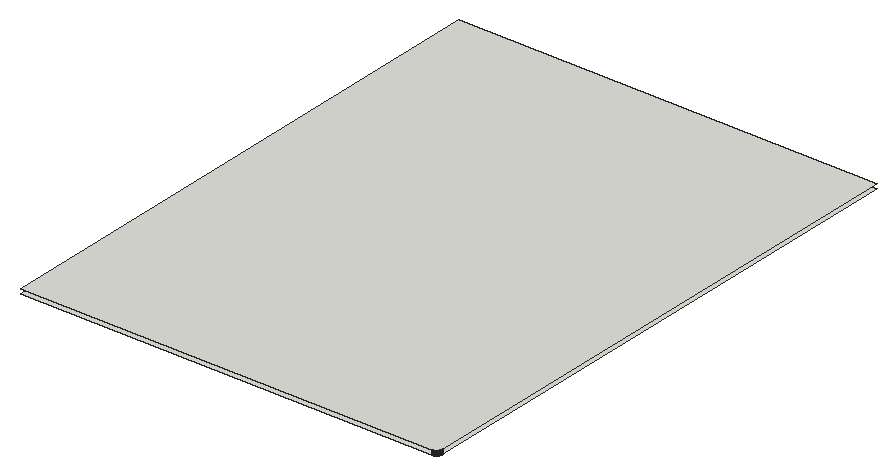
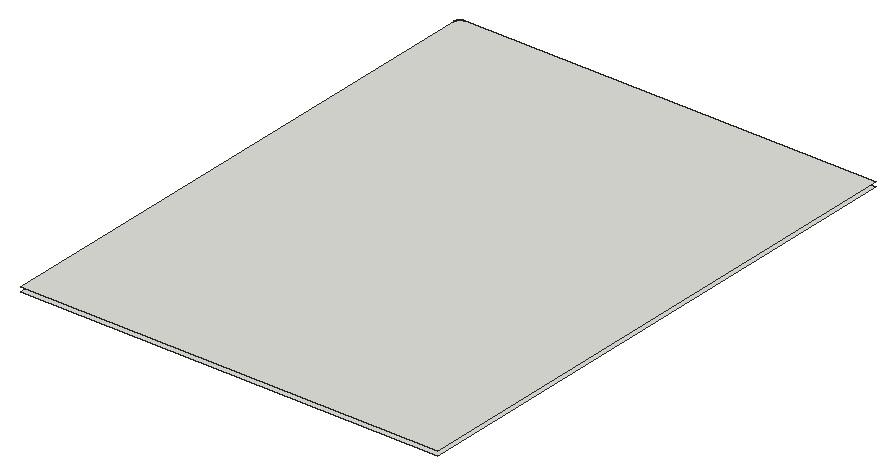
# SketchUp Ruby script. Lengths in inches.
U = 1.inch
M = Sketchup.active_model
def pt(a) = Geom::Point3d.new(a.map { |v| v * U })
def face(e, loops, mat)
  f = e.add_face(loops[0].map { |a| pt(a) })
  loops[1..].each { |l| e.add_face(l.map { |a| pt(a) }).erase! }
  f.material = f.back_material = mat if mat
  f
end
# faces: each face lists its corners as indices into pts; further lists are holes
def faces(e, pts, list, mat = nil) = list.each { |f| face(e, (f[0].is_a?(Array) ? f : [f]).map { |l| l.map { |i| pts[i] } }, mat) }
# xy, xz, yz: faces in a plane at the given z, y or x. An outline is a flat list of corners, or four numbers for a rectangle; further outlines are holes
def ring(l) = l.size == 4 ? [[l[0], l[1]], [l[2], l[1]], [l[2], l[3]], [l[0], l[3]]] : l.each_slice(2).to_a
def flat(e, list, mat, &to3) = list.each { |f| face(e, (f[0].is_a?(Array) ? f : [f]).map { |l| ring(l).map { |u, v| to3.(u, v) } }, mat) }
def xy(e, z, list, mat = nil) = flat(e, list, mat) { |x, y| [x, y, z] }
def xz(e, y, list, mat = nil) = flat(e, list, mat) { |x, z| [x, y, z] }
def yz(e, x, list, mat = nil) = flat(e, list, mat) { |y, z| [x, y, z] }
def lines(e, pts, list) = list.each { |a, b| e.add_line(pt(pts[a]), pt(pts[b])) }
# prism: a flat outline (further loops are holes) pulled along v
def prism(e, loops, v, mat = nil)
  f = face(e, loops, mat); d = Geom::Vector3d.new(v.map { |x| x * U })
  f.pushpull(f.normal.samedirection?(d) ? d.length : -d.length)
end
def box(e, o, s, mat = nil) = prism(e, [[o, [o[0] + s[0], o[1], o[2]], [o[0] + s[0], o[1] + s[1], o[2]], [o[0], o[1] + s[1], o[2]]]], [0, 0, s[2]], mat)
def at(x, y, z, deg = 0) = Geom::Transformation.translation(pt([x, y, z])) * Geom::Transformation.rotation(ORIGIN, Z_AXIS, deg.degrees)
def axes(o, x, y, z) = Geom::Transformation.new([*x, 0, *y, 0, *z, 0, *pt(o).to_a, 1])
def part(name) = M.definitions.add(name)
# library, detail: a bought-in or finely detailed component or shape, given as its bounding box
def library(name, o, s) = part(name).tap { |d| box(d.entities, o, s) }
def detail(e, o, s) = box(e.add_group.entities, o, s)
def put(e, d, t, mat = nil) = e.add_instance(d, t).tap { |i| i.material = mat if mat }
def group(e, t, mat = nil) = e.add_group.tap { |g| g.transformation = t; g.material = mat if mat }.entities
root = M.entities
xy(root,128,[[[48,96,48,600,432,600,432,101.78,431.95,101.23,431.93,101.12,431.92,101.01,431.9,100.9,431.85,100.68,431.83,100.57,431.8,100.46,431.77,100.36,431.74,100.25,431.71,100.15,431.67,100.04,431.63,99.9375,431.59,99.83,431.47,99.53,431.27,99.13,431.21,99.03,431.16,98.9375,431.1,98.84,430.98,98.66,430.92,98.5625,430.85,98.47,430.79,98.38,430.72,98.3,430.65,98.21,430.51,98.04,430.43,97.96,430.36,97.875,430.28,97.8,430.2,97.72,430.125,97.64,430.04,97.57,429.96,97.49,429.79,97.35,429.7,97.28,429.62,97.21,429.53,97.15,429.4375,97.08,429.34,97.02,429.16,96.9,429.0625,96.84,428.97,96.79,428.87,96.73,428.47,96.53,428.17,96.41,428.0625,96.37,427.96,96.33,427.85,96.29,427.75,96.26,427.64,96.23,427.54,96.2,427.43,96.17,427.32,96.15,427.1,96.1,426.99,96.08,426.88,96.07,426.77,96.05,426.22,96],[359.84,432,360.16,432,360.24,432.01,360.3125,432.02,360.39,432.03,360.55,432.05,360.625,432.07,360.7,432.08,360.78,432.1,360.85,432.125,360.93,432.15,361,432.17,361.08,432.2,361.29,432.29,361.36,432.33,361.43,432.36,361.57,432.44,361.63,432.48,361.7,432.53,361.76,432.57,361.83,432.62,362.07,432.82,362.12,432.88,362.18,432.93,362.38,433.17,362.43,433.24,362.47,433.3,362.52,433.37,362.56,433.43,362.64,433.57,362.67,433.64,362.71,433.71,362.8,433.92,362.83,434,362.85,434.07,362.875,434.15,362.9,434.22,362.92,434.3,362.93,434.375,362.95,434.45,362.97,434.61,362.98,434.6875,362.99,434.76,363,434.84,363,435.16,362.99,435.24,362.98,435.3125,362.97,435.39,362.95,435.55,362.93,435.625,362.92,435.7,362.9,435.78,362.875,435.85,362.85,435.93,362.83,436,362.8,436.08,362.71,436.29,362.67,436.36,362.64,436.43,362.56,436.57,362.52,436.63,362.47,436.7,362.43,436.76,362.38,436.83,362.18,437.07,362.12,437.12,362.07,437.18,361.83,437.38,361.76,437.43,361.7,437.47,361.63,437.52,361.57,437.56,361.43,437.64,361.36,437.67,361.29,437.71,361.08,437.8,361,437.83,360.93,437.85,360.85,437.875,360.78,437.9,360.7,437.92,360.625,437.93,360.55,437.95,360.39,437.97,360.3125,437.98,360.24,437.99,360.16,438,359.84,438,359.76,437.99,359.6875,437.98,359.61,437.97,359.45,437.95,359.375,437.93,359.3,437.92,359.22,437.9,359.15,437.875,359.07,437.85,359,437.83,358.92,437.8,358.71,437.71,358.64,437.67,358.57,437.64,358.43,437.56,358.37,437.52,358.3,437.47,358.24,437.43,358.17,437.38,357.93,437.18,357.88,437.12,357.82,437.07,357.62,436.83,357.57,436.76,357.53,436.7,357.48,436.63,357.44,436.57,357.36,436.43,357.33,436.36,357.29,436.29,357.2,436.08,357.17,436,357.15,435.93,357.125,435.85,357.1,435.78,357.08,435.7,357.07,435.625,357.05,435.55,357.03,435.39,357.02,435.3125,357.01,435.24,357,435.16,357,434.84,357.01,434.76,357.02,434.6875,357.03,434.61,357.05,434.45,357.07,434.375,357.08,434.3,357.1,434.22,357.125,434.15,357.15,434.07,357.17,434,357.2,433.92,357.29,433.71,357.33,433.64,357.36,433.57,357.44,433.43,357.48,433.37,357.53,433.3,357.57,433.24,357.62,433.17,357.82,432.93,357.88,432.88,357.93,432.82,358.17,432.62,358.24,432.57,358.3,432.53,358.37,432.48,358.43,432.44,358.57,432.36,358.64,432.33,358.71,432.29,358.92,432.2,359,432.17,359.07,432.15,359.15,432.125,359.22,432.1,359.3,432.08,359.375,432.07,359.45,432.05,359.61,432.03,359.6875,432.02,359.76,432.01],[359.84,525,360.16,525,360.24,525.01,360.3125,525.02,360.39,525.03,360.55,525.05,360.625,525.07,360.7,525.08,360.78,525.1,360.85,525.125,360.93,525.15,361,525.17,361.08,525.2,361.29,525.29,361.36,525.33,361.43,525.36,361.57,525.44,361.63,525.48,361.7,525.53,361.76,525.57,361.83,525.62,362.07,525.82,362.12,525.88,362.18,525.93,362.38,526.17,362.43,526.24,362.47,526.3,362.52,526.37,362.56,526.43,362.64,526.57,362.67,526.64,362.71,526.71,362.8,526.92,362.83,527,362.85,527.07,362.875,527.15,362.9,527.22,362.92,527.3,362.93,527.375,362.95,527.45,362.97,527.61,362.98,527.6875,362.99,527.76,363,527.84,363,528.16,362.99,528.24,362.98,528.3125,362.97,528.39,362.95,528.55,362.93,528.625,362.92,528.7,362.9,528.78,362.875,528.85,362.85,528.93,362.83,529,362.8,529.08,362.71,529.29,362.67,529.36,362.64,529.43,362.56,529.57,362.52,529.63,362.47,529.7,362.43,529.76,362.38,529.83,362.18,530.07,362.12,530.12,362.07,530.18,361.83,530.38,361.76,530.43,361.7,530.47,361.63,530.52,361.57,530.56,361.43,530.64,361.36,530.67,361.29,530.71,361.08,530.8,361,530.83,360.93,530.85,360.85,530.875,360.78,530.9,360.7,530.92,360.625,530.93,360.55,530.95,360.39,530.97,360.3125,530.98,360.24,530.99,360.16,531,359.84,531,359.76,530.99,359.6875,530.98,359.61,530.97,359.45,530.95,359.375,530.93,359.3,530.92,359.22,530.9,359.15,530.875,359.07,530.85,359,530.83,358.92,530.8,358.71,530.71,358.64,530.67,358.57,530.64,358.43,530.56,358.37,530.52,358.3,530.47,358.24,530.43,358.17,530.38,357.93,530.18,357.88,530.12,357.82,530.07,357.62,529.83,357.57,529.76,357.53,529.7,357.48,529.63,357.44,529.57,357.36,529.43,357.33,529.36,357.29,529.29,357.2,529.08,357.17,529,357.15,528.93,357.125,528.85,357.1,528.78,357.08,528.7,357.07,528.625,357.05,528.55,357.03,528.39,357.02,528.3125,357.01,528.24,357,528.16,357,527.84,357.01,527.76,357.02,527.6875,357.03,527.61,357.05,527.45,357.07,527.375,357.08,527.3,357.1,527.22,357.125,527.15,357.15,527.07,357.17,527,357.2,526.92,357.29,526.71,357.33,526.64,357.36,526.57,357.44,526.43,357.48,526.37,357.53,526.3,357.57,526.24,357.62,526.17,357.82,525.93,357.88,525.88,357.93,525.82,358.17,525.62,358.24,525.57,358.3,525.53,358.37,525.48,358.43,525.44,358.57,525.36,358.64,525.33,358.71,525.29,358.92,525.2,359,525.17,359.07,525.15,359.15,525.125,359.22,525.1,359.3,525.08,359.375,525.07,359.45,525.05,359.61,525.03,359.6875,525.02,359.76,525.01],[279.84,525,280.16,525,280.24,525.01,280.3125,525.02,280.39,525.03,280.55,525.05,280.625,525.07,280.7,525.08,280.78,525.1,280.85,525.125,280.93,525.15,281,525.17,281.08,525.2,281.29,525.29,281.36,525.33,281.43,525.36,281.57,525.44,281.63,525.48,281.7,525.53,281.76,525.57,281.83,525.62,282.07,525.82,282.12,525.88,282.18,525.93,282.38,526.17,282.43,526.24,282.47,526.3,282.52,526.37,282.56,526.43,282.64,526.57,282.67,526.64,282.71,526.71,282.8,526.92,282.83,527,282.85,527.07,282.875,527.15,282.9,527.22,282.92,527.3,282.93,527.375,282.95,527.45,282.97,527.61,282.98,527.6875,282.99,527.76,283,527.84,283,528.16,282.99,528.24,282.98,528.3125,282.97,528.39,282.95,528.55,282.93,528.625,282.92,528.7,282.9,528.78,282.875,528.85,282.85,528.93,282.83,529,282.8,529.08,282.71,529.29,282.67,529.36,282.64,529.43,282.56,529.57,282.52,529.63,282.47,529.7,282.43,529.76,282.38,529.83,282.18,530.07,282.12,530.12,282.07,530.18,281.83,530.38,281.76,530.43,281.7,530.47,281.63,530.52,281.57,530.56,281.43,530.64,281.36,530.67,281.29,530.71,281.08,530.8,281,530.83,280.93,530.85,280.85,530.875,280.78,530.9,280.7,530.92,280.625,530.93,280.55,530.95,280.39,530.97,280.3125,530.98,280.24,530.99,280.16,531,279.84,531,279.76,530.99,279.6875,530.98,279.61,530.97,279.45,530.95,279.375,530.93,279.3,530.92,279.22,530.9,279.15,530.875,279.07,530.85,279,530.83,278.92,530.8,278.71,530.71,278.64,530.67,278.57,530.64,278.43,530.56,278.37,530.52,278.3,530.47,278.24,530.43,278.17,530.38,277.93,530.18,277.88,530.12,277.82,530.07,277.62,529.83,277.57,529.76,277.53,529.7,277.48,529.63,277.44,529.57,277.36,529.43,277.33,529.36,277.29,529.29,277.2,529.08,277.17,529,277.15,528.93,277.125,528.85,277.1,528.78,277.08,528.7,277.07,528.625,277.05,528.55,277.03,528.39,277.02,528.3125,277.01,528.24,277,528.16,277,527.84,277.01,527.76,277.02,527.6875,277.03,527.61,277.05,527.45,277.07,527.375,277.08,527.3,277.1,527.22,277.125,527.15,277.15,527.07,277.17,527,277.2,526.92,277.29,526.71,277.33,526.64,277.36,526.57,277.44,526.43,277.48,526.37,277.53,526.3,277.57,526.24,277.62,526.17,277.82,525.93,277.88,525.88,277.93,525.82,278.17,525.62,278.24,525.57,278.3,525.53,278.37,525.48,278.43,525.44,278.57,525.36,278.64,525.33,278.71,525.29,278.92,525.2,279,525.17,279.07,525.15,279.15,525.125,279.22,525.1,279.3,525.08,279.375,525.07,279.45,525.05,279.61,525.03,279.6875,525.02,279.76,525.01],[119.84,153,120.16,153,120.24,153.01,120.3125,153.02,120.39,153.03,120.55,153.05,120.625,153.07,120.7,153.08,120.78,153.1,120.85,153.125,120.93,153.15,121,153.17,121.08,153.2,121.29,153.29,121.36,153.33,121.43,153.36,121.57,153.44,121.63,153.48,121.7,153.53,121.76,153.57,121.83,153.62,122.07,153.82,122.12,153.88,122.18,153.93,122.38,154.17,122.43,154.24,122.47,154.3,122.52,154.37,122.56,154.43,122.64,154.57,122.67,154.64,122.71,154.71,122.8,154.92,122.83,155,122.85,155.07,122.875,155.15,122.9,155.22,122.92,155.3,122.93,155.375,122.95,155.45,122.97,155.61,122.98,155.6875,122.99,155.76,123,155.84,123,156.16,122.99,156.24,122.98,156.3125,122.97,156.39,122.95,156.55,122.93,156.625,122.92,156.7,122.9,156.78,122.875,156.85,122.85,156.93,122.83,157,122.8,157.08,122.71,157.29,122.67,157.36,122.64,157.43,122.56,157.57,122.52,157.63,122.47,157.7,122.43,157.76,122.38,157.83,122.18,158.07,122.12,158.12,122.07,158.18,121.83,158.38,121.76,158.43,121.7,158.47,121.63,158.52,121.57,158.56,121.43,158.64,121.36,158.67,121.29,158.71,121.08,158.8,121,158.83,120.93,158.85,120.85,158.875,120.78,158.9,120.7,158.92,120.625,158.93,120.55,158.95,120.39,158.97,120.3125,158.98,120.24,158.99,120.16,159,119.84,159,119.76,158.99,119.6875,158.98,119.61,158.97,119.45,158.95,119.375,158.93,119.3,158.92,119.22,158.9,119.15,158.875,119.07,158.85,119,158.83,118.92,158.8,118.71,158.71,118.64,158.67,118.57,158.64,118.43,158.56,118.37,158.52,118.3,158.47,118.24,158.43,118.17,158.38,117.93,158.18,117.88,158.12,117.82,158.07,117.62,157.83,117.57,157.76,117.53,157.7,117.48,157.63,117.44,157.57,117.36,157.43,117.33,157.36,117.29,157.29,117.2,157.08,117.17,157,117.15,156.93,117.125,156.85,117.1,156.78,117.08,156.7,117.07,156.625,117.05,156.55,117.03,156.39,117.02,156.3125,117.01,156.24,117,156.16,117,155.84,117.01,155.76,117.02,155.6875,117.03,155.61,117.05,155.45,117.07,155.375,117.08,155.3,117.1,155.22,117.125,155.15,117.15,155.07,117.17,155,117.2,154.92,117.29,154.71,117.33,154.64,117.36,154.57,117.44,154.43,117.48,154.37,117.53,154.3,117.57,154.24,117.62,154.17,117.82,153.93,117.88,153.88,117.93,153.82,118.17,153.62,118.24,153.57,118.3,153.53,118.37,153.48,118.43,153.44,118.57,153.36,118.64,153.33,118.71,153.29,118.92,153.2,119,153.17,119.07,153.15,119.15,153.125,119.22,153.1,119.3,153.08,119.375,153.07,119.45,153.05,119.61,153.03,119.6875,153.02,119.76,153.01],[199.84,153,200.16,153,200.24,153.01,200.3125,153.02,200.39,153.03,200.55,153.05,200.625,153.07,200.7,153.08,200.78,153.1,200.85,153.125,200.93,153.15,201,153.17,201.08,153.2,201.29,153.29,201.36,153.33,201.43,153.36,201.57,153.44,201.63,153.48,201.7,153.53,201.76,153.57,201.83,153.62,202.07,153.82,202.12,153.88,202.18,153.93,202.38,154.17,202.43,154.24,202.47,154.3,202.52,154.37,202.56,154.43,202.64,154.57,202.67,154.64,202.71,154.71,202.8,154.92,202.83,155,202.85,155.07,202.875,155.15,202.9,155.22,202.92,155.3,202.93,155.375,202.95,155.45,202.97,155.61,202.98,155.6875,202.99,155.76,203,155.84,203,156.16,202.99,156.24,202.98,156.3125,202.97,156.39,202.95,156.55,202.93,156.625,202.92,156.7,202.9,156.78,202.875,156.85,202.85,156.93,202.83,157,202.8,157.08,202.71,157.29,202.67,157.36,202.64,157.43,202.56,157.57,202.52,157.63,202.47,157.7,202.43,157.76,202.38,157.83,202.18,158.07,202.12,158.12,202.07,158.18,201.83,158.38,201.76,158.43,201.7,158.47,201.63,158.52,201.57,158.56,201.43,158.64,201.36,158.67,201.29,158.71,201.08,158.8,201,158.83,200.93,158.85,200.85,158.875,200.78,158.9,200.7,158.92,200.625,158.93,200.55,158.95,200.39,158.97,200.3125,158.98,200.24,158.99,200.16,159,199.84,159,199.76,158.99,199.6875,158.98,199.61,158.97,199.45,158.95,199.375,158.93,199.3,158.92,199.22,158.9,199.15,158.875,199.07,158.85,199,158.83,198.92,158.8,198.71,158.71,198.64,158.67,198.57,158.64,198.43,158.56,198.37,158.52,198.3,158.47,198.24,158.43,198.17,158.38,197.93,158.18,197.88,158.12,197.82,158.07,197.62,157.83,197.57,157.76,197.53,157.7,197.48,157.63,197.44,157.57,197.36,157.43,197.33,157.36,197.29,157.29,197.2,157.08,197.17,157,197.15,156.93,197.125,156.85,197.1,156.78,197.08,156.7,197.07,156.625,197.05,156.55,197.03,156.39,197.02,156.3125,197.01,156.24,197,156.16,197,155.84,197.01,155.76,197.02,155.6875,197.03,155.61,197.05,155.45,197.07,155.375,197.08,155.3,197.1,155.22,197.125,155.15,197.15,155.07,197.17,155,197.2,154.92,197.29,154.71,197.33,154.64,197.36,154.57,197.44,154.43,197.48,154.37,197.53,154.3,197.57,154.24,197.62,154.17,197.82,153.93,197.88,153.88,197.93,153.82,198.17,153.62,198.24,153.57,198.3,153.53,198.37,153.48,198.43,153.44,198.57,153.36,198.64,153.33,198.71,153.29,198.92,153.2,199,153.17,199.07,153.15,199.15,153.125,199.22,153.1,199.3,153.08,199.375,153.07,199.45,153.05,199.61,153.03,199.6875,153.02,199.76,153.01],[279.84,153,280.16,153,280.24,153.01,280.3125,153.02,280.39,153.03,280.55,153.05,280.625,153.07,280.7,153.08,280.78,153.1,280.85,153.125,280.93,153.15,281,153.17,281.08,153.2,281.29,153.29,281.36,153.33,281.43,153.36,281.57,153.44,281.63,153.48,281.7,153.53,281.76,153.57,281.83,153.62,282.07,153.82,282.12,153.88,282.18,153.93,282.38,154.17,282.43,154.24,282.47,154.3,282.52,154.37,282.56,154.43,282.64,154.57,282.67,154.64,282.71,154.71,282.8,154.92,282.83,155,282.85,155.07,282.875,155.15,282.9,155.22,282.92,155.3,282.93,155.375,282.95,155.45,282.97,155.61,282.98,155.6875,282.99,155.76,283,155.84,283,156.16,282.99,156.24,282.98,156.3125,282.97,156.39,282.95,156.55,282.93,156.625,282.92,156.7,282.9,156.78,282.875,156.85,282.85,156.93,282.83,157,282.8,157.08,282.71,157.29,282.67,157.36,282.64,157.43,282.56,157.57,282.52,157.63,282.47,157.7,282.43,157.76,282.38,157.83,282.18,158.07,282.12,158.12,282.07,158.18,281.83,158.38,281.76,158.43,281.7,158.47,281.63,158.52,281.57,158.56,281.43,158.64,281.36,158.67,281.29,158.71,281.08,158.8,281,158.83,280.93,158.85,280.85,158.875,280.78,158.9,280.7,158.92,280.625,158.93,280.55,158.95,280.39,158.97,280.3125,158.98,280.24,158.99,280.16,159,279.84,159,279.76,158.99,279.6875,158.98,279.61,158.97,279.45,158.95,279.375,158.93,279.3,158.92,279.22,158.9,279.15,158.875,279.07,158.85,279,158.83,278.92,158.8,278.71,158.71,278.64,158.67,278.57,158.64,278.43,158.56,278.37,158.52,278.3,158.47,278.24,158.43,278.17,158.38,277.93,158.18,277.88,158.12,277.82,158.07,277.62,157.83,277.57,157.76,277.53,157.7,277.48,157.63,277.44,157.57,277.36,157.43,277.33,157.36,277.29,157.29,277.2,157.08,277.17,157,277.15,156.93,277.125,156.85,277.1,156.78,277.08,156.7,277.07,156.625,277.05,156.55,277.03,156.39,277.02,156.3125,277.01,156.24,277,156.16,277,155.84,277.01,155.76,277.02,155.6875,277.03,155.61,277.05,155.45,277.07,155.375,277.08,155.3,277.1,155.22,277.125,155.15,277.15,155.07,277.17,155,277.2,154.92,277.29,154.71,277.33,154.64,277.36,154.57,277.44,154.43,277.48,154.37,277.53,154.3,277.57,154.24,277.62,154.17,277.82,153.93,277.88,153.88,277.93,153.82,278.17,153.62,278.24,153.57,278.3,153.53,278.37,153.48,278.43,153.44,278.57,153.36,278.64,153.33,278.71,153.29,278.92,153.2,279,153.17,279.07,153.15,279.15,153.125,279.22,153.1,279.3,153.08,279.375,153.07,279.45,153.05,279.61,153.03,279.6875,153.02,279.76,153.01],[359.84,153,360.16,153,360.24,153.01,360.3125,153.02,360.39,153.03,360.55,153.05,360.625,153.07,360.7,153.08,360.78,153.1,360.85,153.125,360.93,153.15,361,153.17,361.08,153.2,361.29,153.29,361.36,153.33,361.43,153.36,361.57,153.44,361.63,153.48,361.7,153.53,361.76,153.57,361.83,153.62,362.07,153.82,362.12,153.88,362.18,153.93,362.38,154.17,362.43,154.24,362.47,154.3,362.52,154.37,362.56,154.43,362.64,154.57,362.67,154.64,362.71,154.71,362.8,154.92,362.83,155,362.85,155.07,362.875,155.15,362.9,155.22,362.92,155.3,362.93,155.375,362.95,155.45,362.97,155.61,362.98,155.6875,362.99,155.76,363,155.84,363,156.16,362.99,156.24,362.98,156.3125,362.97,156.39,362.95,156.55,362.93,156.625,362.92,156.7,362.9,156.78,362.875,156.85,362.85,156.93,362.83,157,362.8,157.08,362.71,157.29,362.67,157.36,362.64,157.43,362.56,157.57,362.52,157.63,362.47,157.7,362.43,157.76,362.38,157.83,362.18,158.07,362.12,158.12,362.07,158.18,361.83,158.38,361.76,158.43,361.7,158.47,361.63,158.52,361.57,158.56,361.43,158.64,361.36,158.67,361.29,158.71,361.08,158.8,361,158.83,360.93,158.85,360.85,158.875,360.78,158.9,360.7,158.92,360.625,158.93,360.55,158.95,360.39,158.97,360.3125,158.98,360.24,158.99,360.16,159,359.84,159,359.76,158.99,359.6875,158.98,359.61,158.97,359.45,158.95,359.375,158.93,359.3,158.92,359.22,158.9,359.15,158.875,359.07,158.85,359,158.83,358.92,158.8,358.71,158.71,358.64,158.67,358.57,158.64,358.43,158.56,358.37,158.52,358.3,158.47,358.24,158.43,358.17,158.38,357.93,158.18,357.88,158.12,357.82,158.07,357.62,157.83,357.57,157.76,357.53,157.7,357.48,157.63,357.44,157.57,357.36,157.43,357.33,157.36,357.29,157.29,357.2,157.08,357.17,157,357.15,156.93,357.125,156.85,357.1,156.78,357.08,156.7,357.07,156.625,357.05,156.55,357.03,156.39,357.02,156.3125,357.01,156.24,357,156.16,357,155.84,357.01,155.76,357.02,155.6875,357.03,155.61,357.05,155.45,357.07,155.375,357.08,155.3,357.1,155.22,357.125,155.15,357.15,155.07,357.17,155,357.2,154.92,357.29,154.71,357.33,154.64,357.36,154.57,357.44,154.43,357.48,154.37,357.53,154.3,357.57,154.24,357.62,154.17,357.82,153.93,357.88,153.88,357.93,153.82,358.17,153.62,358.24,153.57,358.3,153.53,358.37,153.48,358.43,153.44,358.57,153.36,358.64,153.33,358.71,153.29,358.92,153.2,359,153.17,359.07,153.15,359.15,153.125,359.22,153.1,359.3,153.08,359.375,153.07,359.45,153.05,359.61,153.03,359.6875,153.02,359.76,153.01],[359.84,246,360.16,246,360.24,246.01,360.3125,246.02,360.39,246.03,360.55,246.05,360.625,246.07,360.7,246.08,360.78,246.1,360.85,246.125,360.93,246.15,361,246.17,361.08,246.2,361.29,246.29,361.36,246.33,361.43,246.36,361.57,246.44,361.63,246.48,361.7,246.53,361.76,246.57,361.83,246.62,362.07,246.82,362.12,246.88,362.18,246.93,362.38,247.17,362.43,247.24,362.47,247.3,362.52,247.37,362.56,247.43,362.64,247.57,362.67,247.64,362.71,247.71,362.8,247.92,362.83,248,362.85,248.07,362.875,248.15,362.9,248.22,362.92,248.3,362.93,248.375,362.95,248.45,362.97,248.61,362.98,248.6875,362.99,248.76,363,248.84,363,249.16,362.99,249.24,362.98,249.3125,362.97,249.39,362.95,249.55,362.93,249.625,362.92,249.7,362.9,249.78,362.875,249.85,362.85,249.93,362.83,250,362.8,250.08,362.71,250.29,362.67,250.36,362.64,250.43,362.56,250.57,362.52,250.63,362.47,250.7,362.43,250.76,362.38,250.83,362.18,251.07,362.12,251.12,362.07,251.18,361.83,251.38,361.76,251.43,361.7,251.47,361.63,251.52,361.57,251.56,361.43,251.64,361.36,251.67,361.29,251.71,361.08,251.8,361,251.83,360.93,251.85,360.85,251.875,360.78,251.9,360.7,251.92,360.625,251.93,360.55,251.95,360.39,251.97,360.3125,251.98,360.24,251.99,360.16,252,359.84,252,359.76,251.99,359.6875,251.98,359.61,251.97,359.45,251.95,359.375,251.93,359.3,251.92,359.22,251.9,359.15,251.875,359.07,251.85,359,251.83,358.92,251.8,358.71,251.71,358.64,251.67,358.57,251.64,358.43,251.56,358.37,251.52,358.3,251.47,358.24,251.43,358.17,251.38,357.93,251.18,357.88,251.12,357.82,251.07,357.62,250.83,357.57,250.76,357.53,250.7,357.48,250.63,357.44,250.57,357.36,250.43,357.33,250.36,357.29,250.29,357.2,250.08,357.17,250,357.15,249.93,357.125,249.85,357.1,249.78,357.08,249.7,357.07,249.625,357.05,249.55,357.03,249.39,357.02,249.3125,357.01,249.24,357,249.16,357,248.84,357.01,248.76,357.02,248.6875,357.03,248.61,357.05,248.45,357.07,248.375,357.08,248.3,357.1,248.22,357.125,248.15,357.15,248.07,357.17,248,357.2,247.92,357.29,247.71,357.33,247.64,357.36,247.57,357.44,247.43,357.48,247.37,357.53,247.3,357.57,247.24,357.62,247.17,357.82,246.93,357.88,246.88,357.93,246.82,358.17,246.62,358.24,246.57,358.3,246.53,358.37,246.48,358.43,246.44,358.57,246.36,358.64,246.33,358.71,246.29,358.92,246.2,359,246.17,359.07,246.15,359.15,246.125,359.22,246.1,359.3,246.08,359.375,246.07,359.45,246.05,359.61,246.03,359.6875,246.02,359.76,246.01],[359.84,339,360.16,339,360.24,339.01,360.3125,339.02,360.39,339.03,360.55,339.05,360.625,339.07,360.7,339.08,360.78,339.1,360.85,339.125,360.93,339.15,361,339.17,361.08,339.2,361.29,339.29,361.36,339.33,361.43,339.36,361.57,339.44,361.63,339.48,361.7,339.53,361.76,339.57,361.83,339.62,362.07,339.82,362.12,339.88,362.18,339.93,362.38,340.17,362.43,340.24,362.47,340.3,362.52,340.37,362.56,340.43,362.64,340.57,362.67,340.64,362.71,340.71,362.8,340.92,362.83,341,362.85,341.07,362.875,341.15,362.9,341.22,362.92,341.3,362.93,341.375,362.95,341.45,362.97,341.61,362.98,341.6875,362.99,341.76,363,341.84,363,342.16,362.99,342.24,362.98,342.3125,362.97,342.39,362.95,342.55,362.93,342.625,362.92,342.7,362.9,342.78,362.875,342.85,362.85,342.93,362.83,343,362.8,343.08,362.71,343.29,362.67,343.36,362.64,343.43,362.56,343.57,362.52,343.63,362.47,343.7,362.43,343.76,362.38,343.83,362.18,344.07,362.12,344.12,362.07,344.18,361.83,344.38,361.76,344.43,361.7,344.47,361.63,344.52,361.57,344.56,361.43,344.64,361.36,344.67,361.29,344.71,361.08,344.8,361,344.83,360.93,344.85,360.85,344.875,360.78,344.9,360.7,344.92,360.625,344.93,360.55,344.95,360.39,344.97,360.3125,344.98,360.24,344.99,360.16,345,359.84,345,359.76,344.99,359.6875,344.98,359.61,344.97,359.45,344.95,359.375,344.93,359.3,344.92,359.22,344.9,359.15,344.875,359.07,344.85,359,344.83,358.92,344.8,358.71,344.71,358.64,344.67,358.57,344.64,358.43,344.56,358.37,344.52,358.3,344.47,358.24,344.43,358.17,344.38,357.93,344.18,357.88,344.12,357.82,344.07,357.62,343.83,357.57,343.76,357.53,343.7,357.48,343.63,357.44,343.57,357.36,343.43,357.33,343.36,357.29,343.29,357.2,343.08,357.17,343,357.15,342.93,357.125,342.85,357.1,342.78,357.08,342.7,357.07,342.625,357.05,342.55,357.03,342.39,357.02,342.3125,357.01,342.24,357,342.16,357,341.84,357.01,341.76,357.02,341.6875,357.03,341.61,357.05,341.45,357.07,341.375,357.08,341.3,357.1,341.22,357.125,341.15,357.15,341.07,357.17,341,357.2,340.92,357.29,340.71,357.33,340.64,357.36,340.57,357.44,340.43,357.48,340.37,357.53,340.3,357.57,340.24,357.62,340.17,357.82,339.93,357.88,339.88,357.93,339.82,358.17,339.62,358.24,339.57,358.3,339.53,358.37,339.48,358.43,339.44,358.57,339.36,358.64,339.33,358.71,339.29,358.92,339.2,359,339.17,359.07,339.15,359.15,339.125,359.22,339.1,359.3,339.08,359.375,339.07,359.45,339.05,359.61,339.03,359.6875,339.02,359.76,339.01]]])
xy(root,132,[[48,96,426.22,96,426.77,96.05,426.88,96.07,426.99,96.08,427.1,96.1,427.32,96.15,427.43,96.17,427.54,96.2,427.64,96.23,427.75,96.26,427.85,96.29,427.96,96.33,428.0625,96.37,428.17,96.41,428.47,96.53,428.87,96.73,428.97,96.79,429.0625,96.84,429.16,96.9,429.34,97.02,429.4375,97.08,429.53,97.15,429.62,97.21,429.7,97.28,429.79,97.35,429.96,97.49,430.04,97.57,430.125,97.64,430.2,97.72,430.28,97.8,430.36,97.875,430.43,97.96,430.51,98.04,430.65,98.21,430.72,98.3,430.79,98.38,430.85,98.47,430.92,98.5625,430.98,98.66,431.1,98.84,431.16,98.9375,431.21,99.03,431.27,99.13,431.47,99.53,431.59,99.83,431.63,99.9375,431.67,100.04,431.71,100.15,431.74,100.25,431.77,100.36,431.8,100.46,431.83,100.57,431.85,100.68,431.9,100.9,431.92,101.01,431.93,101.12,431.95,101.23,432,101.78,432,600,48,600]])
xz(root,96,[[426,128,426.11,132],[426.11,128,426.22,132]])
xz(root,153,[[359.84,128,359.92,129],[359.92,128,360,129],[360,128,360.08,129],[360.08,128,360.16,129]])
yz(root,432,[[101.78,128,101.89,132],[101.89,128,102,132]])
p = [[426.33,96.01,132],[426.22,96,132],[426.22,96,128],[426.33,96.01,128],[426.44,96.02,132],[426.44,96.02,128],
  [426.55,96.03,132],[426.55,96.03,128],[426.66,96.04,132],[426.66,96.04,128],[426.77,96.05,132],[426.77,96.05,128],
  [426.88,96.07,132],[426.88,96.07,128],[426.99,96.08,132],[426.99,96.08,128],[427.1,96.1,132],[427.1,96.1,128],
  [427.21,96.125,132],[427.21,96.125,128],[427.32,96.15,132],[427.32,96.15,128],[427.43,96.17,132],[427.43,96.17,128],
  [427.54,96.2,132],[427.54,96.2,128],[427.64,96.23,132],[427.64,96.23,128],[427.75,96.26,132],[427.75,96.26,128],
  [427.85,96.29,132],[427.85,96.29,128],[427.96,96.33,132],[427.96,96.33,128],[428.0625,96.37,132],[428.0625,96.37,128],
  [428.17,96.41,132],[428.17,96.41,128],[428.27,96.45,132],[428.27,96.45,128],[428.37,96.49,132],[428.37,96.49,128],
  [428.47,96.53,132],[428.47,96.53,128],[428.57,96.58,132],[428.57,96.58,128],[428.67,96.63,132],[428.67,96.63,128],
  [428.77,96.68,132],[428.77,96.68,128],[428.87,96.73,132],[428.87,96.73,128],[428.97,96.79,132],[428.97,96.79,128],
  [429.0625,96.84,132],[429.0625,96.84,128],[429.16,96.9,132],[429.16,96.9,128],[429.25,96.96,132],[429.25,96.96,128],
  [429.34,97.02,132],[429.34,97.02,128],[429.4375,97.08,132],[429.4375,97.08,128],[429.53,97.15,132],[429.53,97.15,128],
  [429.62,97.21,132],[429.62,97.21,128],[429.7,97.28,132],[429.7,97.28,128],[429.79,97.35,132],[429.79,97.35,128],
  [429.875,97.42,132],[429.875,97.42,128],[429.96,97.49,132],[429.96,97.49,128],[430.04,97.57,132],[430.04,97.57,128],
  [430.125,97.64,132],[430.125,97.64,128],[430.2,97.72,132],[430.2,97.72,128],[430.28,97.8,132],[430.28,97.8,128],
  [430.36,97.875,132],[430.36,97.875,128],[430.43,97.96,132],[430.43,97.96,128],[430.51,98.04,132],[430.51,98.04,128],
  [430.58,98.125,132],[430.58,98.125,128],[430.65,98.21,132],[430.65,98.21,128],[430.72,98.3,132],[430.72,98.3,128],
  [430.79,98.38,132],[430.79,98.38,128],[430.85,98.47,132],[430.85,98.47,128],[430.92,98.5625,132],[430.92,98.5625,128],
  [430.98,98.66,132],[430.98,98.66,128],[431.04,98.75,132],[431.04,98.75,128],[431.1,98.84,132],[431.1,98.84,128],
  [431.16,98.9375,132],[431.16,98.9375,128],[431.21,99.03,132],[431.21,99.03,128],[431.27,99.13,132],[431.27,99.13,128],
  [431.32,99.23,132],[431.32,99.23,128],[431.37,99.33,132],[431.37,99.33,128],[431.42,99.43,132],[431.42,99.43,128],
  [431.47,99.53,132],[431.47,99.53,128],[431.51,99.63,132],[431.51,99.63,128],[431.55,99.73,132],[431.55,99.73,128],
  [431.59,99.83,132],[431.59,99.83,128],[431.63,99.9375,132],[431.63,99.9375,128],[431.67,100.04,132],[431.67,100.04,128],
  [431.71,100.15,132],[431.71,100.15,128],[431.74,100.25,132],[431.74,100.25,128],[431.77,100.36,132],[431.77,100.36,128],
  [431.8,100.46,132],[431.8,100.46,128],[431.83,100.57,132],[431.83,100.57,128],[431.85,100.68,132],[431.85,100.68,128],
  [431.875,100.79,132],[431.875,100.79,128],[431.9,100.9,132],[431.9,100.9,128],[431.92,101.01,132],[431.92,101.01,128],
  [431.93,101.12,132],[431.93,101.12,128],[431.95,101.23,132],[431.95,101.23,128],[431.96,101.34,132],[431.96,101.34,128],
  [431.97,101.45,132],[431.97,101.45,128],[431.98,101.56,132],[431.98,101.56,128],[431.99,101.67,132],[431.99,101.67,128],
  [432,101.78,132],[432,101.78,128],[359.6875,153.02,128],[359.61,153.03,128],[359.61,153.03,129],[359.6875,153.02,129],
  [359.76,153.01,128],[359.76,153.01,129],[359.84,153,128],[359.84,153,129],[360.24,153.01,128],[360.16,153,128],
  [360.16,153,129],[360.24,153.01,129],[360.3125,153.02,128],[360.3125,153.02,129],[360.39,153.03,128],[360.39,153.03,129],
  [360.47,153.04,128],[360.47,153.04,129],[360.55,153.05,128],[360.55,153.05,129],[360.625,153.07,128],[360.625,153.07,129],
  [360.7,153.08,128],[360.7,153.08,129],[360.78,153.1,128],[360.78,153.1,129],[360.85,153.125,128],[360.85,153.125,129],
  [360.93,153.15,128],[360.93,153.15,129],[361,153.17,128],[361,153.17,129],[361.08,153.2,128],[361.08,153.2,129],
  [361.15,153.23,128],[361.15,153.23,129],[361.22,153.26,128],[361.22,153.26,129],[361.29,153.29,128],[361.29,153.29,129],
  [361.36,153.33,128],[361.36,153.33,129],[361.43,153.36,128],[361.43,153.36,129],[361.5,153.4,128],[361.5,153.4,129],
  [361.57,153.44,128],[361.57,153.44,129],[361.63,153.48,128],[361.63,153.48,129],[361.7,153.53,128],[361.7,153.53,129],
  [361.76,153.57,128],[361.76,153.57,129],[361.83,153.62,128],[361.83,153.62,129],[361.89,153.67,128],[361.89,153.67,129],
  [361.95,153.72,128],[361.95,153.72,129],[362.01,153.77,128],[362.01,153.77,129],[362.07,153.82,128],[362.07,153.82,129],
  [362.12,153.88,128],[362.12,153.88,129],[362.18,153.93,128],[362.18,153.93,129],[362.23,153.99,128],[362.23,153.99,129],
  [362.28,154.05,128],[362.28,154.05,129],[362.33,154.11,128],[362.33,154.11,129],[362.38,154.17,128],[362.38,154.17,129],
  [362.43,154.24,128],[362.43,154.24,129],[362.47,154.3,128],[362.47,154.3,129],[362.52,154.37,128],[362.52,154.37,129],
  [362.56,154.43,128],[362.56,154.43,129],[362.6,154.5,128],[362.6,154.5,129],[362.64,154.57,128],[362.64,154.57,129],
  [362.67,154.64,128],[362.67,154.64,129],[362.71,154.71,128],[362.71,154.71,129],[362.74,154.78,128],[362.74,154.78,129],
  [362.77,154.85,128],[362.77,154.85,129],[362.8,154.92,128],[362.8,154.92,129],[362.83,155,128],[362.83,155,129],
  [362.85,155.07,128],[362.85,155.07,129],[362.875,155.15,128],[362.875,155.15,129],[362.9,155.22,128],[362.9,155.22,129],
  [362.92,155.3,128],[362.92,155.3,129],[362.93,155.375,128],[362.93,155.375,129],[362.95,155.45,128],[362.95,155.45,129],
  [362.96,155.53,128],[362.96,155.53,129],[362.97,155.61,128],[362.97,155.61,129],[362.98,155.6875,128],[362.98,155.6875,129],
  [362.99,155.76,128],[362.99,155.76,129]]
faces(root,p,[[0,1,2,3],[4,0,3,5],[6,4,5,7],[8,6,7,9],[10,8,9,11],[12,10,11,13],[14,12,13,15],[16,14,15,17],
  [18,16,17,19],[20,18,19,21],[22,20,21,23],[24,22,23,25],[26,24,25,27],[28,26,27,29],[30,28,29,31],[32,30,31,33],
  [34,32,33,35],[36,34,35,37],[38,36,37,39],[40,38,39,41],[42,40,41,43],[44,42,43,45],[46,44,45,47],[48,46,47,49],
  [50,48,49,51],[52,50,51,53],[54,52,53,55],[56,54,55,57],[58,56,57,59],[60,58,59,61],[62,60,61,63],[64,62,63,65],
  [66,64,65,67],[68,66,67,69],[70,68,69,71],[72,70,71,73],[74,72,73,75],[76,74,75,77],[78,76,77,79],[80,78,79,81],
  [82,80,81,83],[84,82,83,85],[86,84,85,87],[88,86,87,89],[90,88,89,91],[92,90,91,93],[94,92,93,95],[96,94,95,97],
  [98,96,97,99],[100,98,99,101],[102,100,101,103],[104,102,103,105],[106,104,105,107],[108,106,107,109],[110,108,109,111],[112,110,111,113],
  [114,112,113,115],[116,114,115,117],[118,116,117,119],[120,118,119,121],[122,120,121,123],[124,122,123,125],[126,124,125,127],[128,126,127,129],
  [130,128,129,131],[132,130,131,133],[134,132,133,135],[136,134,135,137],[138,136,137,139],[140,138,139,141],[142,140,141,143],[144,142,143,145],
  [146,144,145,147],[148,146,147,149],[150,148,149,151],[152,150,151,153],[154,152,153,155],[156,154,155,157],[158,156,157,159],[160,158,159,161],
  [162,160,161,163],[164,165,166,167],[168,164,167,169],[170,168,169,171],[172,173,174,175],[176,172,175,177],[178,176,177,179],[180,178,179,181],
  [182,180,181,183],[184,182,183,185],[186,184,185,187],[188,186,187,189],[190,188,189,191],[192,190,191,193],[194,192,193,195],[196,194,195,197],
  [198,196,197,199],[200,198,199,201],[202,200,201,203],[204,202,203,205],[206,204,205,207],[208,206,207,209],[210,208,209,211],[212,210,211,213],
  [214,212,213,215],[216,214,215,217],[218,216,217,219],[220,218,219,221],[222,220,221,223],[224,222,223,225],[226,224,225,227],[228,226,227,229],
  [230,228,229,231],[232,230,231,233],[234,232,233,235],[236,234,235,237],[238,236,237,239],[240,238,239,241],[242,240,241,243],[244,242,243,245],
  [246,244,245,247],[248,246,247,249],[250,248,249,251],[252,250,251,253],[254,252,253,255],[256,254,255,257],[258,256,257,259],[260,258,259,261],
  [262,260,261,263],[264,262,263,265],[266,264,265,267],[268,266,267,269],[270,268,269,271],[272,270,271,273],[274,272,273,275],[276,274,275,277],
  [278,276,277,279],[280,278,279,281],[282,280,281,283]])
